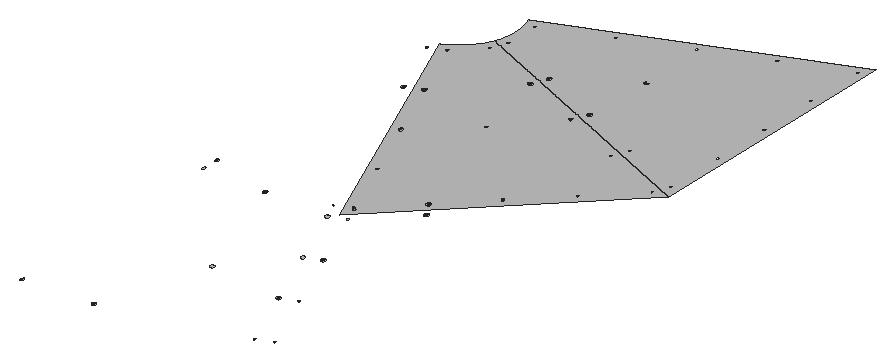
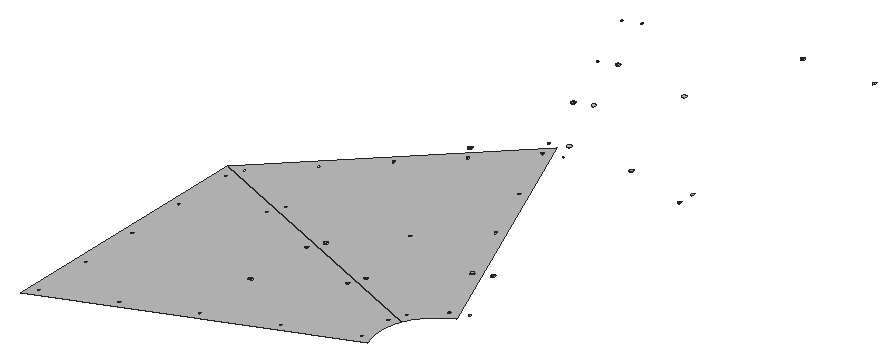
# SketchUp Ruby script. Lengths in inches.
U = 1.inch
M = Sketchup.active_model
def pt(a) = Geom::Point3d.new(a.map { |v| v * U })
def face(e, loops, mat)
  f = e.add_face(loops[0].map { |a| pt(a) })
  loops[1..].each { |l| e.add_face(l.map { |a| pt(a) }).erase! }
  f.material = f.back_material = mat if mat
  f
end
# faces: each face lists its corners as indices into pts; further lists are holes
def faces(e, pts, list, mat = nil) = list.each { |f| face(e, (f[0].is_a?(Array) ? f : [f]).map { |l| l.map { |i| pts[i] } }, mat) }
# xy, xz, yz: faces in a plane at the given z, y or x. An outline is a flat list of corners, or four numbers for a rectangle; further outlines are holes
def ring(l) = l.size == 4 ? [[l[0], l[1]], [l[2], l[1]], [l[2], l[3]], [l[0], l[3]]] : l.each_slice(2).to_a
def flat(e, list, mat, &to3) = list.each { |f| face(e, (f[0].is_a?(Array) ? f : [f]).map { |l| ring(l).map { |u, v| to3.(u, v) } }, mat) }
def xy(e, z, list, mat = nil) = flat(e, list, mat) { |x, y| [x, y, z] }
def xz(e, y, list, mat = nil) = flat(e, list, mat) { |x, z| [x, y, z] }
def yz(e, x, list, mat = nil) = flat(e, list, mat) { |y, z| [x, y, z] }
def lines(e, pts, list) = list.each { |a, b| e.add_line(pt(pts[a]), pt(pts[b])) }
# prism: a flat outline (further loops are holes) pulled along v
def prism(e, loops, v, mat = nil)
  f = face(e, loops, mat); d = Geom::Vector3d.new(v.map { |x| x * U })
  f.pushpull(f.normal.samedirection?(d) ? d.length : -d.length)
end
def box(e, o, s, mat = nil) = prism(e, [[o, [o[0] + s[0], o[1], o[2]], [o[0] + s[0], o[1] + s[1], o[2]], [o[0], o[1] + s[1], o[2]]]], [0, 0, s[2]], mat)
def at(x, y, z, deg = 0) = Geom::Transformation.translation(pt([x, y, z])) * Geom::Transformation.rotation(ORIGIN, Z_AXIS, deg.degrees)
def axes(o, x, y, z) = Geom::Transformation.new([*x, 0, *y, 0, *z, 0, *pt(o).to_a, 1])
def part(name) = M.definitions.add(name)
# library, detail: a bought-in or finely detailed component or shape, given as its bounding box
def library(name, o, s) = part(name).tap { |d| box(d.entities, o, s) }
def detail(e, o, s) = box(e.add_group.entities, o, s)
def put(e, d, t, mat = nil) = e.add_instance(d, t).tap { |i| i.material = mat if mat }
def group(e, t, mat = nil) = e.add_group.tap { |g| g.transformation = t; g.material = mat if mat }.entities
root = M.entities
M.materials.add("[Metal_Steel_Textured_White]").color = [191, 191, 191]
xy(root,3.625,[[149.818,137.074,149.818,137.125,149.827,137.127,149.836,137.13,149.844,137.136,149.85,137.144,149.853,137.153,149.854,137.162,149.853,137.172,149.85,137.18,149.844,137.188,149.836,137.194,149.827,137.197,149.818,137.199,149.818,137.25,149.841,137.247,149.862,137.238,149.88,137.224,149.894,137.206,149.903,137.185,149.906,137.162,149.903,137.139,149.894,137.118,149.88,137.1,149.862,137.086,149.841,137.077],[149.818,137.125,149.818,137.142,149.823,137.143,149.828,137.145,149.832,137.148,149.835,137.152,149.837,137.157,149.838,137.162,149.837,137.167,149.835,137.172,149.832,137.176,149.828,137.179,149.823,137.181,149.818,137.182,149.818,137.199,149.827,137.197,149.836,137.194,149.844,137.188,149.85,137.18,149.853,137.172,149.854,137.162,149.853,137.153,149.85,137.144,149.844,137.136,149.836,137.13,149.827,137.127],[[153.108,137.28,153.085,137.283,153.063,137.292,153.045,137.306,153.031,137.325,153.022,137.346,153.019,137.369,153.022,137.392,153.031,137.414,153.045,137.432,153.063,137.446,153.085,137.455,153.108,137.458,153.131,137.455,153.152,137.446,153.171,137.432,153.185,137.414,153.194,137.392,153.197,137.369,153.194,137.346,153.185,137.325,153.171,137.306,153.152,137.292,153.131,137.283],[153.108,137.281,153.13,137.284,153.152,137.293,153.17,137.307,153.184,137.325,153.193,137.347,153.196,137.369,153.193,137.392,153.184,137.413,153.17,137.432,153.152,137.445,153.13,137.454,153.108,137.457,153.085,137.454,153.064,137.445,153.046,137.432,153.032,137.413,153.023,137.392,153.02,137.369,153.023,137.347,153.032,137.325,153.046,137.307,153.064,137.293,153.085,137.284]],[[153.108,137.281,153.085,137.284,153.064,137.293,153.046,137.307,153.032,137.325,153.023,137.347,153.02,137.369,153.023,137.392,153.032,137.413,153.046,137.432,153.064,137.445,153.085,137.454,153.108,137.457,153.13,137.454,153.152,137.445,153.17,137.432,153.184,137.413,153.193,137.392,153.196,137.369,153.193,137.347,153.184,137.325,153.17,137.307,153.152,137.293,153.13,137.284],[153.108,137.333,153.117,137.334,153.126,137.338,153.134,137.343,153.139,137.351,153.143,137.36,153.144,137.369,153.143,137.379,153.139,137.388,153.134,137.395,153.126,137.401,153.117,137.405,153.108,137.406,153.098,137.405,153.089,137.401,153.082,137.395,153.076,137.388,153.072,137.379,153.071,137.369,153.072,137.36,153.076,137.351,153.082,137.343,153.089,137.338,153.098,137.334]],[[159.48,138.971,159.471,138.972,159.462,138.976,159.454,138.982,159.448,138.989,159.445,138.998,159.443,139.008,159.445,139.017,159.448,139.026,159.454,139.034,159.462,139.039,159.471,139.043,159.48,139.044,159.49,139.043,159.498,139.039,159.506,139.034,159.512,139.026,159.515,139.017,159.517,139.008,159.515,138.998,159.512,138.989,159.506,138.982,159.498,138.976,159.49,138.972],[159.475,138.988,159.485,138.988,159.49,138.99,159.494,138.994,159.497,138.998,159.499,139.002,159.5,139.008,159.499,139.013,159.497,139.018,159.494,139.022,159.49,139.025,159.485,139.027,159.48,139.028,159.475,139.027,159.47,139.025,159.466,139.022,159.463,139.018,159.461,139.013,159.46,139.008,159.461,139.002,159.463,138.998,159.466,138.994,159.47,138.99]],
  [159.475,138.988,159.47,138.99,159.466,138.994,159.463,138.998,159.461,139.002,159.46,139.008,159.461,139.013,159.463,139.018,159.466,139.022,159.47,139.025,159.475,139.027,159.48,139.028,159.485,139.027,159.49,139.025,159.494,139.022,159.497,139.018,159.499,139.013,159.5,139.008,159.499,139.002,159.497,138.998,159.494,138.994,159.49,138.99,159.485,138.988],[[160.218,139.277,160.208,139.278,160.199,139.282,160.192,139.287,160.186,139.295,160.182,139.304,160.181,139.313,160.182,139.323,160.186,139.331,160.192,139.339,160.199,139.345,160.208,139.349,160.218,139.35,160.227,139.349,160.236,139.345,160.244,139.339,160.249,139.331,160.253,139.323,160.254,139.313,160.253,139.304,160.249,139.295,160.244,139.287,160.236,139.282,160.227,139.278],[160.218,139.293,160.223,139.294,160.228,139.296,160.232,139.299,160.235,139.303,160.237,139.308,160.238,139.313,160.237,139.318,160.235,139.323,160.232,139.327,160.228,139.33,160.223,139.332,160.218,139.333,160.213,139.332,160.208,139.33,160.204,139.327,160.2,139.323,160.198,139.318,160.198,139.308,160.2,139.303,160.204,139.299,160.208,139.296,160.213,139.294]],[160.218,139.293,160.213,139.294,160.208,139.296,160.204,139.299,160.2,139.303,160.198,139.308,160.198,139.318,160.2,139.323,160.204,139.327,160.208,139.33,160.213,139.332,160.218,139.333,160.223,139.332,160.228,139.33,160.232,139.327,160.235,139.323,160.237,139.318,160.238,139.313,160.237,139.308,160.235,139.303,160.232,139.299,160.228,139.296,160.223,139.294],[[158.237,141.919,158.214,141.922,158.193,141.931,158.175,141.945,158.16,141.963,158.152,141.985,158.149,142.008,158.152,142.031,158.16,142.052,158.175,142.07,158.193,142.085,158.214,142.093,158.237,142.096,158.26,142.093,158.282,142.085,158.3,142.07,158.314,142.052,158.323,142.031,158.326,142.008,158.323,141.985,158.314,141.963,158.3,141.945,158.282,141.931,158.26,141.922],[158.237,141.92,158.26,141.923,158.281,141.931,158.3,141.945,158.314,141.964,158.322,141.985,158.325,142.008,158.322,142.03,158.314,142.052,158.3,142.07,158.281,142.084,158.26,142.093,158.237,142.096,158.215,142.093,158.193,142.084,158.175,142.07,158.161,142.052,158.153,142.03,158.15,142.008,158.153,141.985,158.161,141.964,158.175,141.945,158.193,141.931,158.215,141.923]],[[158.237,141.971,158.228,141.972,158.219,141.976,158.212,141.982,158.206,141.989,158.202,141.998,158.201,142.008,158.202,142.017,158.206,142.026,158.212,142.033,158.219,142.039,158.228,142.043,158.237,142.044,158.247,142.043,158.256,142.039,158.263,142.033,158.269,142.026,158.273,142.017,158.274,142.008,158.273,141.998,158.269,141.989,158.263,141.982,158.256,141.976,158.247,141.972],[158.232,141.988,158.243,141.988,158.247,141.99,158.252,141.993,158.255,141.998,158.257,142.002,158.257,142.013,158.255,142.018,158.252,142.022,158.247,142.025,158.243,142.027,158.237,142.028,158.232,142.027,158.227,142.025,158.223,142.022,158.22,142.018,158.218,142.013,158.217,142.008,158.218,142.002,158.22,141.998,158.223,141.993,158.227,141.99]],
  [158.232,141.988,158.227,141.99,158.223,141.993,158.22,141.998,158.218,142.002,158.217,142.008,158.218,142.013,158.22,142.018,158.223,142.022,158.227,142.025,158.232,142.027,158.237,142.028,158.243,142.027,158.247,142.025,158.252,142.022,158.255,142.018,158.257,142.013,158.257,142.002,158.255,141.998,158.252,141.993,158.247,141.99,158.243,141.988],[[154.784,142.264,154.761,142.267,154.74,142.276,154.722,142.29,154.708,142.308,154.699,142.329,154.696,142.352,154.699,142.375,154.708,142.396,154.722,142.414,154.74,142.428,154.761,142.437,154.784,142.44,154.807,142.437,154.828,142.428,154.846,142.414,154.86,142.396,154.869,142.375,154.872,142.352,154.869,142.329,154.86,142.308,154.846,142.29,154.828,142.276,154.807,142.267],[154.784,142.315,154.794,142.317,154.802,142.32,154.81,142.326,154.816,142.334,154.819,142.342,154.821,142.352,154.819,142.361,154.816,142.37,154.81,142.378,154.802,142.384,154.794,142.387,154.784,142.389,154.775,142.387,154.766,142.384,154.758,142.378,154.752,142.37,154.749,142.361,154.747,142.352,154.749,142.342,154.752,142.334,154.758,142.326,154.766,142.32,154.775,142.317]],[[158.975,142.277,158.966,142.278,158.957,142.281,158.949,142.287,158.943,142.295,158.94,142.304,158.939,142.313,158.94,142.323,158.943,142.331,158.949,142.339,158.957,142.345,158.966,142.349,158.975,142.35,158.985,142.349,158.993,142.345,159.001,142.339,159.007,142.331,159.01,142.323,159.012,142.313,159.01,142.304,159.007,142.295,159.001,142.287,158.993,142.281,158.985,142.278],[158.975,142.293,158.98,142.294,158.985,142.296,158.989,142.299,158.992,142.303,158.994,142.308,158.995,142.313,158.994,142.318,158.992,142.323,158.989,142.327,158.985,142.33,158.98,142.332,158.975,142.333,158.97,142.332,158.965,142.33,158.961,142.327,158.958,142.323,158.956,142.318,158.955,142.313,158.956,142.308,158.958,142.303,158.961,142.299,158.965,142.296,158.97,142.294]],[158.975,142.293,158.97,142.294,158.965,142.296,158.961,142.299,158.958,142.303,158.956,142.308,158.955,142.313,158.956,142.318,158.958,142.323,158.961,142.327,158.965,142.33,158.97,142.332,158.975,142.333,158.98,142.332,158.985,142.33,158.989,142.327,158.992,142.323,158.994,142.318,158.995,142.313,158.994,142.308,158.992,142.303,158.989,142.299,158.985,142.296,158.98,142.294],[[156.995,144.92,156.972,144.923,156.951,144.931,156.933,144.945,156.919,144.964,156.91,144.985,156.907,145.008,156.91,145.03,156.919,145.052,156.933,145.07,156.951,145.084,156.972,145.092,156.995,145.095,157.018,145.092,157.039,145.084,157.057,145.07,157.071,145.052,157.08,145.03,157.083,145.008,157.08,144.985,157.071,144.964,157.057,144.945,157.039,144.931,157.018,144.923],[156.995,144.971,157.004,144.972,157.013,144.976,157.021,144.982,157.027,144.989,157.03,144.998,157.031,145.008,157.03,145.017,157.027,145.026,157.021,145.033,157.013,145.039,157.004,145.043,156.995,145.044,156.985,145.043,156.977,145.039,156.969,145.033,156.963,145.026,156.959,145.017,156.958,145.008,156.959,144.998,156.963,144.989,156.969,144.982,156.977,144.976,156.985,144.972]],
  [[157.732,145.224,157.709,145.227,157.688,145.236,157.67,145.25,157.656,145.269,157.647,145.29,157.644,145.313,157.647,145.336,157.656,145.358,157.67,145.376,157.688,145.39,157.709,145.399,157.732,145.402,157.755,145.399,157.777,145.39,157.795,145.376,157.809,145.358,157.818,145.336,157.821,145.313,157.818,145.29,157.809,145.269,157.795,145.25,157.777,145.236,157.755,145.227],[157.732,145.225,157.755,145.228,157.776,145.237,157.795,145.251,157.809,145.269,157.817,145.29,157.82,145.313,157.817,145.336,157.809,145.357,157.795,145.375,157.776,145.389,157.755,145.398,157.732,145.401,157.71,145.398,157.689,145.389,157.67,145.375,157.656,145.357,157.648,145.336,157.645,145.313,157.648,145.29,157.656,145.269,157.67,145.251,157.689,145.237,157.71,145.228]],[[157.732,145.277,157.723,145.278,157.714,145.281,157.707,145.287,157.701,145.295,157.697,145.304,157.696,145.313,157.697,145.323,157.701,145.331,157.707,145.339,157.714,145.345,157.723,145.348,157.732,145.35,157.742,145.348,157.751,145.345,157.758,145.339,157.764,145.331,157.768,145.323,157.769,145.313,157.768,145.304,157.764,145.295,157.758,145.287,157.751,145.281,157.742,145.278],[157.732,145.293,157.738,145.294,157.742,145.296,157.747,145.299,157.75,145.303,157.752,145.308,157.752,145.318,157.75,145.323,157.747,145.327,157.742,145.33,157.738,145.332,157.732,145.333,157.727,145.332,157.723,145.33,157.718,145.327,157.715,145.323,157.713,145.318,157.713,145.308,157.715,145.303,157.718,145.299,157.723,145.296,157.727,145.294]],[157.732,145.293,157.727,145.294,157.723,145.296,157.718,145.299,157.715,145.303,157.713,145.308,157.713,145.318,157.715,145.323,157.718,145.327,157.723,145.33,157.727,145.332,157.732,145.333,157.738,145.332,157.742,145.33,157.747,145.327,157.75,145.323,157.752,145.318,157.752,145.308,157.75,145.303,157.747,145.299,157.742,145.296,157.738,145.294],[[152.785,147.919,152.762,147.922,152.741,147.931,152.722,147.945,152.708,147.963,152.699,147.985,152.696,148.008,152.699,148.031,152.708,148.052,152.722,148.07,152.741,148.085,152.762,148.093,152.785,148.096,152.808,148.093,152.829,148.085,152.848,148.07,152.862,148.052,152.871,148.031,152.874,148.008,152.871,147.985,152.862,147.963,152.848,147.945,152.829,147.931,152.808,147.922],[152.785,147.92,152.808,147.923,152.829,147.931,152.847,147.945,152.861,147.964,152.87,147.985,152.873,148.008,152.87,148.03,152.861,148.051,152.847,148.07,152.829,148.084,152.808,148.092,152.785,148.095,152.762,148.092,152.741,148.084,152.723,148.07,152.709,148.051,152.7,148.03,152.697,148.008,152.7,147.985,152.709,147.964,152.723,147.945,152.741,147.931,152.762,147.923]],[[155.752,147.919,155.729,147.922,155.708,147.931,155.689,147.945,155.675,147.963,155.666,147.985,155.663,148.008,155.666,148.031,155.675,148.052,155.689,148.07,155.708,148.085,155.729,148.093,155.752,148.096,155.775,148.093,155.797,148.085,155.815,148.07,155.829,148.052,155.838,148.031,155.841,148.008,155.838,147.985,155.829,147.963,155.815,147.945,155.797,147.931,155.775,147.922],[155.752,147.92,155.775,147.923,155.796,147.931,155.814,147.945,155.828,147.964,155.837,147.985,155.84,148.008,155.837,148.03,155.828,148.051,155.814,148.07,155.796,148.084,155.775,148.092,155.752,148.095,155.729,148.092,155.708,148.084,155.69,148.07,155.676,148.051,155.667,148.03,155.664,148.008,155.667,147.985,155.676,147.964,155.69,147.945,155.708,147.931,155.729,147.923]],
  [149.818,147.92,149.818,147.971,149.827,147.972,149.836,147.976,149.844,147.982,149.85,147.989,149.853,147.998,149.854,148.008,149.853,148.017,149.85,148.026,149.844,148.033,149.836,148.039,149.827,148.043,149.818,148.044,149.818,148.095,149.841,148.092,149.862,148.084,149.88,148.07,149.894,148.051,149.903,148.03,149.906,148.008,149.903,147.985,149.894,147.964,149.88,147.945,149.862,147.931,149.841,147.923],[[152.785,147.92,152.762,147.923,152.741,147.931,152.723,147.945,152.709,147.964,152.7,147.985,152.697,148.008,152.7,148.03,152.709,148.051,152.723,148.07,152.741,148.084,152.762,148.092,152.785,148.095,152.808,148.092,152.829,148.084,152.847,148.07,152.861,148.051,152.87,148.03,152.873,148.008,152.87,147.985,152.861,147.964,152.847,147.945,152.829,147.931,152.808,147.923],[152.785,147.971,152.795,147.972,152.803,147.976,152.811,147.982,152.817,147.989,152.82,147.998,152.822,148.008,152.82,148.017,152.817,148.026,152.811,148.033,152.803,148.039,152.795,148.043,152.785,148.044,152.776,148.043,152.767,148.039,152.759,148.033,152.753,148.026,152.75,148.017,152.748,148.008,152.75,147.998,152.753,147.989,152.759,147.982,152.767,147.976,152.776,147.972]],[[155.752,147.92,155.729,147.923,155.708,147.931,155.69,147.945,155.676,147.964,155.667,147.985,155.664,148.008,155.667,148.03,155.676,148.051,155.69,148.07,155.708,148.084,155.729,148.092,155.752,148.095,155.775,148.092,155.796,148.084,155.814,148.07,155.828,148.051,155.837,148.03,155.84,148.008,155.837,147.985,155.828,147.964,155.814,147.945,155.796,147.931,155.775,147.923],[155.752,147.971,155.762,147.972,155.771,147.976,155.778,147.982,155.784,147.989,155.788,147.998,155.789,148.008,155.788,148.017,155.784,148.026,155.778,148.033,155.771,148.039,155.762,148.043,155.752,148.044,155.743,148.043,155.734,148.039,155.726,148.033,155.721,148.026,155.717,148.017,155.716,148.008,155.717,147.998,155.721,147.989,155.726,147.982,155.734,147.976,155.743,147.972]],[[156.49,148.276,156.48,148.278,156.472,148.281,156.464,148.287,156.458,148.295,156.455,148.304,156.453,148.313,156.455,148.323,156.458,148.331,156.464,148.339,156.472,148.345,156.48,148.348,156.49,148.35,156.499,148.348,156.508,148.345,156.516,148.339,156.522,148.331,156.525,148.323,156.526,148.313,156.525,148.304,156.522,148.295,156.516,148.287,156.508,148.281,156.499,148.278],[156.49,148.293,156.495,148.294,156.5,148.296,156.504,148.299,156.507,148.303,156.509,148.308,156.51,148.313,156.509,148.318,156.507,148.323,156.504,148.327,156.5,148.33,156.495,148.332,156.49,148.333,156.485,148.332,156.48,148.33,156.476,148.327,156.473,148.323,156.471,148.318,156.47,148.313,156.471,148.308,156.473,148.303,156.476,148.299,156.48,148.296,156.485,148.294]],[156.49,148.293,156.485,148.294,156.48,148.296,156.476,148.299,156.473,148.303,156.471,148.308,156.47,148.313,156.471,148.318,156.473,148.323,156.476,148.327,156.48,148.33,156.485,148.332,156.49,148.333,156.495,148.332,156.5,148.33,156.504,148.327,156.507,148.323,156.509,148.318,156.51,148.313,156.509,148.308,156.507,148.303,156.504,148.299,156.5,148.296,156.495,148.294],
  [[156.019,148.407,150.836,160.919,150.995,160.99,151.149,161.073,151.297,161.165,151.438,161.266,151.573,161.376,151.7,161.495,151.819,161.623,151.929,161.757,152.031,161.899,152.123,162.047,152.205,162.2,152.277,162.359,164.789,157.176],[152.551,157.734,152.574,157.737,152.595,157.746,152.614,157.76,152.628,157.778,152.637,157.8,152.64,157.823,152.637,157.846,152.628,157.867,152.614,157.886,152.595,157.9,152.574,157.909,152.551,157.912,152.528,157.909,152.506,157.9,152.488,157.886,152.474,157.867,152.465,157.846,152.462,157.823,152.465,157.8,152.474,157.778,152.488,157.76,152.506,157.746,152.528,157.737],[164.084,156.947,164.107,156.95,164.128,156.959,164.147,156.973,164.161,156.992,164.17,157.013,164.173,157.036,164.17,157.059,164.161,157.081,164.147,157.099,164.128,157.113,164.107,157.122,164.084,157.125,164.061,157.122,164.039,157.113,164.021,157.099,164.007,157.081,163.998,157.059,163.995,157.036,163.998,157.013,164.007,156.992,164.021,156.973,164.039,156.959,164.061,156.95],[158.14,151.004,158.163,151.007,158.185,151.016,158.203,151.03,158.217,151.048,158.226,151.07,158.229,151.093,158.226,151.116,158.217,151.137,158.203,151.156,158.185,151.17,158.163,151.179,158.14,151.182,158.117,151.179,158.096,151.17,158.077,151.156,158.063,151.137,158.054,151.116,158.051,151.093,158.054,151.07,158.063,151.048,158.077,151.03,158.096,151.016,158.117,151.007],[156.122,156.984,156.145,156.987,156.167,156.996,156.185,157.01,156.199,157.029,156.208,157.05,156.211,157.073,156.208,157.096,156.199,157.117,156.185,157.136,156.167,157.15,156.145,157.159,156.122,157.162,156.099,157.159,156.078,157.15,156.06,157.136,156.045,157.117,156.037,157.096,156.033,157.073,156.037,157.05,156.045,157.029,156.06,157.01,156.078,156.996,156.099,156.987],[155.372,160.556,155.395,160.559,155.417,160.568,155.435,160.582,155.449,160.6,155.458,160.622,155.461,160.645,155.458,160.668,155.449,160.689,155.435,160.707,155.417,160.722,155.395,160.73,155.372,160.733,155.349,160.73,155.328,160.722,155.31,160.707,155.295,160.689,155.287,160.668,155.284,160.645,155.287,160.622,155.295,160.6,155.31,160.582,155.328,160.568,155.349,160.559],[158.276,159.353,158.299,159.356,158.321,159.365,158.339,159.379,158.353,159.397,158.362,159.419,158.365,159.442,158.362,159.465,158.353,159.486,158.339,159.505,158.321,159.519,158.299,159.528,158.276,159.531,158.253,159.528,158.232,159.519,158.213,159.505,158.199,159.486,158.19,159.465,158.1875,159.442,158.19,159.419,158.199,159.397,158.213,159.379,158.232,159.365,158.253,159.356],[156.159,149.023,156.182,149.026,156.204,149.035,156.222,149.049,156.236,149.067,156.245,149.088,156.248,149.112,156.245,149.135,156.236,149.156,156.222,149.174,156.204,149.188,156.182,149.197,156.159,149.2,156.136,149.197,156.115,149.188,156.096,149.174,156.082,149.156,156.073,149.135,156.07,149.112,156.073,149.088,156.082,149.067,156.096,149.049,156.115,149.035,156.136,149.026],[162.103,154.966,162.126,154.969,162.147,154.978,162.165,154.992,162.18,155.011,162.189,155.032,162.192,155.055,162.189,155.078,162.18,155.099,162.165,155.118,162.147,155.132,162.126,155.141,162.103,155.144,162.08,155.141,162.058,155.132,162.04,155.118,162.026,155.099,162.017,155.078,162.014,155.055,162.017,155.032,162.026,155.011,162.04,154.992,162.058,154.978,162.08,154.969],[152.469,161.758,152.492,161.761,152.513,161.77,152.532,161.784,152.546,161.803,152.555,161.824,152.558,161.847,152.555,161.87,152.546,161.892,152.532,161.91,152.513,161.924,152.492,161.933,152.469,161.936,152.446,161.933,152.424,161.924,152.406,161.91,152.392,161.892,152.383,161.87,152.38,161.847,152.383,161.824,152.392,161.803,152.406,161.784,152.424,161.77,152.446,161.761],[161.18,158.15,161.203,158.153,161.224,158.162,161.243,158.176,161.257,158.195,161.266,158.216,161.269,158.239,161.266,158.262,161.257,158.283,161.243,158.302,161.224,158.316,161.203,158.325,161.18,158.328,161.157,158.325,161.136,158.316,161.117,158.302,161.103,158.283,161.094,158.262,161.091,158.239,161.094,158.216,161.103,158.195,161.117,158.176,161.136,158.162,161.157,158.153],[154.956,151.926,154.979,151.929,155.001,151.938,155.019,151.952,155.033,151.971,155.042,151.992,155.045,152.015,155.042,152.038,155.033,152.06,155.019,152.078,155.001,152.092,154.979,152.101,154.956,152.104,154.933,152.101,154.912,152.092,154.893,152.078,154.879,152.06,154.87,152.038,154.867,152.015,154.87,151.992,154.879,151.971,154.893,151.952,154.912,151.938,154.933,151.929],[160.121,152.985,160.144,152.988,160.166,152.997,160.184,153.011,160.198,153.029,160.207,153.051,160.21,153.074,160.207,153.097,160.198,153.118,160.184,153.137,160.166,153.151,160.144,153.16,160.121,153.163,160.098,153.16,160.077,153.151,160.059,153.137,160.044,153.118,160.036,153.097,160.033,153.074,160.036,153.051,160.044,153.029,160.059,153.011,160.077,152.997,160.098,152.988],[151.348,160.638,151.371,160.641,151.392,160.65,151.411,160.664,151.425,160.682,151.434,160.704,151.437,160.727,151.434,160.75,151.425,160.771,151.411,160.79,151.392,160.804,151.371,160.8125,151.348,160.816,151.325,160.8125,151.304,160.804,151.285,160.79,151.271,160.771,151.262,160.75,151.259,160.727,151.262,160.704,151.271,160.682,151.285,160.664,151.304,160.65,151.325,160.641],[153.754,154.83,153.777,154.833,153.798,154.842,153.816,154.856,153.831,154.875,153.839,154.896,153.842,154.919,153.839,154.942,153.831,154.964,153.816,154.982,153.798,154.996,153.777,155.005,153.754,155.008,153.731,155.005,153.709,154.996,153.691,154.982,153.677,154.964,153.668,154.942,153.665,154.919,153.668,154.896,153.677,154.875,153.691,154.856,153.709,154.842,153.731,154.833]],[149.818,148.718,149.818,148.769,149.827,148.771,149.836,148.774,149.844,148.78,149.85,148.788,149.853,148.796,149.854,148.806,149.853,148.815,149.85,148.824,149.844,148.832,149.836,148.838,149.827,148.841,149.818,148.843,149.818,148.894,149.841,148.891,149.862,148.882,149.88,148.868,149.894,148.85,149.903,148.829,149.906,148.806,149.903,148.783,149.894,148.762,149.88,148.744,149.862,148.73,149.841,148.721],[149.818,148.769,149.818,148.786,149.823,148.787,149.828,148.789,149.832,148.792,149.835,148.796,149.837,148.801,149.838,148.806,149.837,148.811,149.835,148.816,149.832,148.82,149.828,148.823,149.823,148.825,149.818,148.826,149.818,148.843,149.827,148.841,149.836,148.838,149.844,148.832,149.85,148.824,149.853,148.815,149.854,148.806,149.853,148.796,149.85,148.788,149.844,148.78,149.836,148.774,149.827,148.771],[149.818,148.786,149.818,148.826,149.823,148.825,149.828,148.823,149.832,148.82,149.835,148.816,149.837,148.811,149.838,148.806,149.837,148.801,149.835,148.796,149.832,148.792,149.828,148.789,149.823,148.787],[155.421,148.786,155.416,148.787,155.412,148.789,155.407,148.792,155.404,148.796,155.402,148.801,155.402,148.811,155.404,148.816,155.407,148.82,155.412,148.823,155.416,148.825,155.421,148.826,155.427,148.825,155.431,148.823,155.436,148.82,155.439,148.816,155.441,148.811,155.441,148.801,155.439,148.796,155.436,148.792,155.431,148.789,155.427,148.787],
  [[156.159,149.023,156.136,149.026,156.115,149.035,156.096,149.049,156.082,149.067,156.073,149.088,156.07,149.112,156.073,149.135,156.082,149.156,156.096,149.174,156.115,149.188,156.136,149.197,156.159,149.2,156.182,149.197,156.204,149.188,156.222,149.174,156.236,149.156,156.245,149.135,156.248,149.112,156.245,149.088,156.236,149.067,156.222,149.049,156.204,149.035,156.182,149.026],[156.159,149.024,156.182,149.027,156.203,149.035,156.221,149.049,156.235,149.068,156.244,149.089,156.247,149.112,156.244,149.134,156.235,149.155,156.221,149.174,156.203,149.1875,156.182,149.196,156.159,149.199,156.136,149.196,156.115,149.1875,156.097,149.174,156.083,149.155,156.074,149.134,156.071,149.112,156.074,149.089,156.083,149.068,156.097,149.049,156.115,149.035,156.136,149.027]],[[156.159,149.075,156.15,149.076,156.141,149.08,156.133,149.086,156.127,149.093,156.124,149.102,156.123,149.112,156.124,149.121,156.127,149.13,156.133,149.137,156.141,149.143,156.15,149.147,156.159,149.148,156.169,149.147,156.177,149.143,156.185,149.137,156.191,149.13,156.194,149.121,156.196,149.112,156.194,149.102,156.191,149.093,156.185,149.086,156.177,149.08,156.169,149.076],[156.154,149.092,156.164,149.092,156.169,149.094,156.173,149.097,156.176,149.102,156.178,149.106,156.179,149.112,156.178,149.117,156.176,149.121,156.173,149.126,156.169,149.129,156.164,149.131,156.154,149.131,156.149,149.129,156.145,149.126,156.142,149.121,156.14,149.117,156.139,149.112,156.14,149.106,156.142,149.102,156.145,149.097,156.149,149.094]],[156.154,149.092,156.149,149.094,156.145,149.097,156.142,149.102,156.14,149.106,156.139,149.112,156.14,149.117,156.142,149.121,156.145,149.126,156.149,149.129,156.154,149.131,156.164,149.131,156.169,149.129,156.173,149.126,156.176,149.121,156.178,149.117,156.179,149.112,156.178,149.106,156.176,149.102,156.173,149.097,156.169,149.094,156.164,149.092],[[158.588,150.322,158.565,150.325,158.544,150.334,158.525,150.348,158.511,150.367,158.502,150.388,158.499,150.411,158.502,150.434,158.511,150.456,158.525,150.474,158.544,150.488,158.565,150.497,158.588,150.5,158.611,150.497,158.632,150.488,158.651,150.474,158.665,150.456,158.674,150.434,158.677,150.411,158.674,150.388,158.665,150.367,158.651,150.348,158.632,150.334,158.611,150.325],[158.588,150.323,158.611,150.326,158.632,150.335,158.65,150.349,158.664,150.367,158.673,150.388,158.676,150.411,158.673,150.434,158.664,150.455,158.65,150.473,158.632,150.487,158.611,150.496,158.588,150.499,158.565,150.496,158.544,150.487,158.526,150.473,158.512,150.455,158.503,150.434,158.5,150.411,158.503,150.388,158.512,150.367,158.526,150.349,158.544,150.335,158.565,150.326]],[[158.588,150.375,158.578,150.376,158.57,150.379,158.562,150.385,158.556,150.393,158.553,150.402,158.551,150.411,158.553,150.421,158.556,150.429,158.562,150.437,158.57,150.443,158.578,150.447,158.588,150.448,158.597,150.447,158.606,150.443,158.614,150.437,158.62,150.429,158.623,150.421,158.625,150.411,158.623,150.402,158.62,150.393,158.614,150.385,158.606,150.379,158.597,150.376],[158.588,150.391,158.593,150.392,158.598,150.394,158.602,150.397,158.605,150.401,158.607,150.406,158.608,150.411,158.607,150.416,158.605,150.421,158.602,150.425,158.598,150.428,158.593,150.43,158.588,150.431,158.583,150.43,158.578,150.428,158.574,150.425,158.571,150.421,158.569,150.416,158.568,150.411,158.569,150.406,158.571,150.401,158.574,150.397,158.578,150.394,158.583,150.392]],
  [158.588,150.391,158.583,150.392,158.578,150.394,158.574,150.397,158.571,150.401,158.569,150.406,158.568,150.411,158.569,150.416,158.571,150.421,158.574,150.425,158.578,150.428,158.583,150.43,158.588,150.431,158.593,150.43,158.598,150.428,158.602,150.425,158.605,150.421,158.607,150.416,158.608,150.411,158.607,150.406,158.605,150.401,158.602,150.397,158.598,150.394,158.593,150.392],[[158.14,151.004,158.117,151.007,158.096,151.016,158.077,151.03,158.063,151.048,158.054,151.07,158.051,151.093,158.054,151.116,158.063,151.137,158.077,151.156,158.096,151.17,158.117,151.179,158.14,151.182,158.163,151.179,158.185,151.17,158.203,151.156,158.217,151.137,158.226,151.116,158.229,151.093,158.226,151.07,158.217,151.048,158.203,151.03,158.185,151.016,158.163,151.007],[158.14,151.005,158.163,151.008,158.184,151.017,158.202,151.03,158.216,151.049,158.225,151.07,158.228,151.093,158.225,151.115,158.216,151.137,158.202,151.155,158.184,151.169,158.163,151.178,158.14,151.181,158.118,151.178,158.096,151.169,158.078,151.155,158.064,151.137,158.055,151.115,158.052,151.093,158.055,151.07,158.064,151.049,158.078,151.03,158.096,151.017,158.118,151.008]],[[158.14,151.056,158.131,151.057,158.122,151.061,158.114,151.067,158.109,151.074,158.105,151.083,158.104,151.093,158.105,151.102,158.109,151.111,158.114,151.119,158.122,151.124,158.131,151.128,158.14,151.129,158.15,151.128,158.159,151.124,158.166,151.119,158.172,151.111,158.176,151.102,158.177,151.093,158.176,151.083,158.172,151.074,158.166,151.067,158.159,151.061,158.15,151.057],[158.135,151.073,158.145,151.073,158.15,151.075,158.158,151.083,158.16,151.088,158.16,151.098,158.158,151.103,158.154,151.107,158.15,151.11,158.145,151.112,158.14,151.113,158.135,151.112,158.13,151.11,158.126,151.107,158.123,151.103,158.121,151.098,158.12,151.093,158.121,151.088,158.123,151.083,158.126,151.079,158.13,151.075]],[158.135,151.073,158.13,151.075,158.126,151.079,158.123,151.083,158.121,151.088,158.12,151.093,158.121,151.098,158.123,151.103,158.126,151.107,158.13,151.11,158.135,151.112,158.14,151.113,158.145,151.112,158.15,151.11,158.154,151.107,158.158,151.103,158.16,151.098,158.16,151.088,158.158,151.083,158.15,151.075,158.145,151.073],[[154.956,151.979,154.947,151.98,154.938,151.984,154.93,151.989,154.925,151.997,154.921,152.006,154.92,152.015,154.921,152.025,154.925,152.034,154.93,152.041,154.938,152.047,154.947,152.051,154.956,152.052,154.966,152.051,154.975,152.047,154.982,152.041,154.988,152.034,154.992,152.025,154.993,152.015,154.992,152.006,154.988,151.997,154.982,151.989,154.975,151.984,154.966,151.98],[154.956,151.995,154.962,151.996,154.966,151.998,154.97,152.001,154.974,152.005,154.976,152.01,154.976,152.02,154.974,152.025,154.966,152.033,154.962,152.035,154.951,152.035,154.946,152.033,154.942,152.029,154.939,152.025,154.937,152.02,154.936,152.015,154.937,152.01,154.939,152.005,154.942,152.001,154.946,151.998,154.951,151.996]],
  [154.956,151.995,154.951,151.996,154.946,151.998,154.942,152.001,154.939,152.005,154.937,152.01,154.936,152.015,154.937,152.02,154.939,152.025,154.942,152.029,154.946,152.033,154.951,152.035,154.962,152.035,154.966,152.033,154.974,152.025,154.976,152.02,154.976,152.01,154.974,152.005,154.97,152.001,154.966,151.998,154.962,151.996],[[160.121,152.985,160.098,152.988,160.077,152.997,160.059,153.011,160.044,153.029,160.036,153.051,160.033,153.074,160.036,153.097,160.044,153.118,160.059,153.137,160.077,153.151,160.098,153.16,160.121,153.163,160.144,153.16,160.166,153.151,160.184,153.137,160.198,153.118,160.207,153.097,160.21,153.074,160.207,153.051,160.198,153.029,160.184,153.011,160.166,152.997,160.144,152.988],[160.121,152.986,160.144,152.989,160.165,152.998,160.184,153.012,160.198,153.03,160.206,153.051,160.209,153.074,160.206,153.097,160.198,153.118,160.184,153.136,160.165,153.15,160.144,153.159,160.121,153.162,160.099,153.159,160.078,153.15,160.059,153.136,160.045,153.118,160.037,153.097,160.034,153.074,160.037,153.051,160.045,153.03,160.059,153.012,160.078,152.998,160.099,152.989]],[[160.121,153.037,160.112,153.038,160.103,153.042,160.096,153.048,160.09,153.056,160.086,153.064,160.085,153.074,160.086,153.083,160.09,153.092,160.096,153.1,160.103,153.106,160.112,153.109,160.121,153.11,160.131,153.109,160.14,153.106,160.147,153.1,160.153,153.092,160.157,153.083,160.158,153.074,160.157,153.064,160.153,153.056,160.147,153.048,160.14,153.042,160.131,153.038],[160.121,153.054,160.127,153.055,160.131,153.057,160.136,153.06,160.139,153.064,160.141,153.069,160.141,153.079,160.139,153.084,160.136,153.088,160.131,153.091,160.127,153.093,160.121,153.094,160.116,153.093,160.111,153.091,160.107,153.088,160.104,153.084,160.102,153.079,160.102,153.069,160.104,153.064,160.107,153.06,160.111,153.057,160.116,153.055]],[160.121,153.054,160.116,153.055,160.111,153.057,160.107,153.06,160.104,153.064,160.102,153.069,160.102,153.079,160.104,153.084,160.107,153.088,160.111,153.091,160.116,153.093,160.121,153.094,160.127,153.093,160.131,153.091,160.136,153.088,160.139,153.084,160.141,153.079,160.141,153.069,160.139,153.064,160.136,153.06,160.131,153.057,160.127,153.055],[[153.754,154.831,153.731,154.834,153.71,154.843,153.691,154.857,153.677,154.875,153.669,154.896,153.666,154.919,153.669,154.942,153.677,154.963,153.691,154.981,153.71,154.995,153.731,155.004,153.754,155.007,153.776,155.004,153.798,154.995,153.816,154.981,153.83,154.963,153.838,154.942,153.841,154.919,153.838,154.896,153.83,154.875,153.816,154.857,153.798,154.843,153.776,154.834],[153.754,154.882,153.763,154.884,153.772,154.887,153.779,154.893,153.785,154.901,153.789,154.91,153.79,154.919,153.789,154.929,153.785,154.9375,153.779,154.945,153.772,154.951,153.763,154.954,153.754,154.956,153.744,154.954,153.735,154.951,153.728,154.945,153.722,154.9375,153.718,154.929,153.717,154.919,153.718,154.91,153.722,154.901,153.728,154.893,153.735,154.887,153.744,154.884]],
  [[153.754,154.882,153.744,154.884,153.735,154.887,153.728,154.893,153.722,154.901,153.718,154.91,153.717,154.919,153.718,154.929,153.722,154.9375,153.728,154.945,153.735,154.951,153.744,154.954,153.754,154.956,153.763,154.954,153.772,154.951,153.779,154.945,153.785,154.9375,153.789,154.929,153.79,154.919,153.789,154.91,153.785,154.901,153.779,154.893,153.772,154.887,153.763,154.884],[153.754,154.899,153.759,154.9,153.764,154.902,153.768,154.905,153.771,154.909,153.773,154.914,153.774,154.919,153.773,154.924,153.771,154.929,153.768,154.933,153.764,154.936,153.759,154.938,153.754,154.939,153.748,154.938,153.744,154.936,153.739,154.933,153.736,154.929,153.734,154.924,153.734,154.914,153.736,154.909,153.739,154.905,153.744,154.902,153.748,154.9]],[[164.789,157.176,152.277,162.359,152.338,162.522,152.389,162.689,152.428,162.858,152.457,163.03,152.474,163.203,152.479,163.377,152.474,163.551,152.457,163.725,152.428,163.897,152.389,164.066,152.338,164.233,152.277,164.396,164.789,169.578],[152.774,162.496,152.797,162.499,152.819,162.508,152.837,162.522,152.851,162.541,152.86,162.562,152.863,162.585,152.86,162.608,152.851,162.629,152.837,162.648,152.819,162.662,152.797,162.671,152.774,162.674,152.751,162.671,152.73,162.662,152.711,162.648,152.697,162.629,152.688,162.608,152.685,162.585,152.688,162.562,152.697,162.541,152.711,162.522,152.73,162.508,152.751,162.499],[164.389,160.487,164.412,160.49,164.434,160.499,164.452,160.513,164.466,160.531,164.475,160.553,164.478,160.576,164.475,160.599,164.466,160.62,164.452,160.638,164.434,160.653,164.412,160.661,164.389,160.665,164.366,160.661,164.345,160.653,164.327,160.638,164.3125,160.62,164.303,160.599,164.3,160.576,164.303,160.553,164.3125,160.531,164.327,160.513,164.345,160.499,164.366,160.49],[158.734,163.289,158.757,163.292,158.778,163.3,158.797,163.315,158.811,163.333,158.82,163.354,158.823,163.377,158.82,163.4,158.811,163.422,158.797,163.44,158.778,163.454,158.757,163.463,158.734,163.466,158.711,163.463,158.689,163.454,158.671,163.44,158.657,163.422,158.648,163.4,158.645,163.377,158.648,163.354,158.657,163.333,158.671,163.315,158.689,163.3,158.711,163.292],[158.582,166.487,158.605,166.49,158.626,166.498,158.645,166.513,158.659,166.531,158.668,166.552,158.671,166.575,158.668,166.598,158.659,166.62,158.645,166.638,158.626,166.652,158.605,166.661,158.582,166.664,158.559,166.661,158.537,166.652,158.519,166.638,158.505,166.62,158.496,166.598,158.493,166.575,158.496,166.552,158.505,166.531,158.519,166.513,158.537,166.498,158.559,166.49],[155.678,161.293,155.701,161.296,155.722,161.305,155.741,161.319,155.755,161.338,155.764,161.359,155.767,161.382,155.764,161.405,155.755,161.427,155.741,161.445,155.722,161.459,155.701,161.468,155.678,161.471,155.655,161.468,155.634,161.459,155.615,161.445,155.601,161.427,155.592,161.405,155.589,161.382,155.592,161.359,155.601,161.338,155.615,161.319,155.634,161.305,155.655,161.296],[164.389,166.09,164.412,166.093,164.434,166.102,164.452,166.116,164.466,166.135,164.475,166.156,164.478,166.179,164.475,166.202,164.466,166.224,164.452,166.242,164.434,166.256,164.412,166.265,164.389,166.268,164.366,166.265,164.345,166.256,164.327,166.242,164.3125,166.224,164.303,166.202,164.3,166.179,164.303,166.156,164.3125,166.135,164.327,166.116,164.345,166.102,164.366,166.093],[152.774,164.081,152.797,164.084,152.819,164.093,152.837,164.107,152.851,164.125,152.86,164.147,152.863,164.17,152.86,164.193,152.851,164.214,152.837,164.233,152.819,164.247,152.797,164.256,152.774,164.259,152.751,164.256,152.73,164.247,152.711,164.233,152.697,164.214,152.688,164.193,152.685,164.17,152.688,164.147,152.697,164.125,152.711,164.107,152.73,164.093,152.751,164.084],[158.582,160.091,158.605,160.094,158.626,160.102,158.645,160.117,158.659,160.135,158.668,160.156,158.671,160.179,158.668,160.202,158.659,160.224,158.645,160.242,158.626,160.256,158.605,160.265,158.582,160.268,158.559,160.265,158.537,160.256,158.519,160.242,158.505,160.224,158.496,160.202,158.493,160.179,158.496,160.156,158.505,160.135,158.519,160.117,158.537,160.102,158.559,160.094],[164.389,163.289,164.412,163.292,164.434,163.3,164.452,163.315,164.466,163.333,164.475,163.354,164.478,163.377,164.475,163.4,164.466,163.422,164.452,163.44,164.434,163.454,164.412,163.463,164.389,163.466,164.366,163.463,164.345,163.454,164.327,163.44,164.3125,163.422,164.303,163.4,164.3,163.377,164.303,163.354,164.3125,163.333,164.327,163.315,164.345,163.3,164.366,163.292],[161.486,167.689,161.509,167.692,161.53,167.701,161.548,167.715,161.5625,167.734,161.571,167.755,161.574,167.778,161.571,167.801,161.5625,167.823,161.548,167.841,161.53,167.855,161.509,167.864,161.486,167.867,161.463,167.864,161.441,167.855,161.423,167.841,161.409,167.823,161.4,167.801,161.397,167.778,161.4,167.755,161.409,167.734,161.423,167.715,161.441,167.701,161.463,167.692],[155.678,165.284,155.701,165.287,155.722,165.296,155.741,165.31,155.755,165.328,155.764,165.35,155.767,165.373,155.764,165.396,155.755,165.417,155.741,165.435,155.722,165.45,155.701,165.459,155.678,165.462,155.655,165.459,155.634,165.45,155.615,165.435,155.601,165.417,155.592,165.396,155.589,165.373,155.592,165.35,155.601,165.328,155.615,165.31,155.634,165.296,155.655,165.287],[164.389,168.892,164.412,168.895,164.434,168.904,164.452,168.918,164.466,168.937,164.475,168.958,164.478,168.981,164.475,169.004,164.466,169.025,164.452,169.044,164.434,169.058,164.412,169.067,164.389,169.07,164.366,169.067,164.345,169.058,164.327,169.044,164.3125,169.025,164.303,169.004,164.3,168.981,164.303,168.958,164.3125,168.937,164.327,168.918,164.345,168.904,164.366,168.895],[164.389,157.685,164.412,157.688,164.434,157.697,164.452,157.711,164.466,157.729,164.475,157.751,164.478,157.774,164.475,157.797,164.466,157.818,164.452,157.837,164.434,157.851,164.412,157.86,164.389,157.863,164.366,157.86,164.345,157.851,164.327,157.837,164.3125,157.818,164.303,157.797,164.3,157.774,164.303,157.751,164.3125,157.729,164.327,157.711,164.345,157.697,164.366,157.688],[161.486,158.888,161.509,158.891,161.53,158.9,161.548,158.914,161.5625,158.932,161.571,158.954,161.574,158.977,161.571,159,161.5625,159.021,161.548,159.039,161.53,159.054,161.509,159.0625,161.486,159.066,161.463,159.0625,161.441,159.054,161.423,159.039,161.409,159.021,161.4,159,161.397,158.977,161.4,158.954,161.409,158.932,161.423,158.914,161.441,158.9,161.463,158.891]],[[151.813,157.428,151.79,157.431,151.769,157.44,151.75,157.454,151.736,157.473,151.727,157.494,151.724,157.517,151.727,157.54,151.736,157.562,151.75,157.58,151.769,157.594,151.79,157.603,151.813,157.606,151.836,157.603,151.858,157.594,151.876,157.58,151.89,157.562,151.899,157.54,151.902,157.517,151.899,157.494,151.89,157.473,151.876,157.454,151.858,157.44,151.836,157.431],[151.813,157.429,151.836,157.432,151.857,157.441,151.875,157.455,151.889,157.473,151.898,157.495,151.901,157.517,151.898,157.54,151.889,157.561,151.875,157.579,151.857,157.593,151.836,157.602,151.813,157.605,151.79,157.602,151.769,157.593,151.751,157.579,151.737,157.561,151.728,157.54,151.725,157.517,151.728,157.495,151.737,157.473,151.751,157.455,151.769,157.441,151.79,157.432]],[[151.813,157.429,151.79,157.432,151.769,157.441,151.751,157.455,151.737,157.473,151.728,157.495,151.725,157.517,151.728,157.54,151.737,157.561,151.751,157.579,151.769,157.593,151.79,157.602,151.813,157.605,151.836,157.602,151.857,157.593,151.875,157.579,151.889,157.561,151.898,157.54,151.901,157.517,151.898,157.495,151.889,157.473,151.875,157.455,151.857,157.441,151.836,157.432],[151.813,157.481,151.823,157.482,151.831,157.486,151.839,157.491,151.845,157.499,151.848,157.508,151.85,157.517,151.848,157.527,151.845,157.536,151.839,157.543,151.831,157.549,151.823,157.553,151.813,157.554,151.804,157.553,151.795,157.549,151.787,157.543,151.781,157.536,151.778,157.527,151.777,157.517,151.778,157.508,151.781,157.499,151.787,157.491,151.795,157.486,151.804,157.482]],[[151.813,157.481,151.804,157.482,151.795,157.486,151.787,157.491,151.781,157.499,151.778,157.508,151.777,157.517,151.778,157.527,151.781,157.536,151.787,157.543,151.795,157.549,151.804,157.553,151.813,157.554,151.823,157.553,151.831,157.549,151.839,157.543,151.845,157.536,151.848,157.527,151.85,157.517,151.848,157.508,151.845,157.499,151.839,157.491,151.831,157.486,151.823,157.482],[151.813,157.497,151.818,157.498,151.823,157.5,151.827,157.503,151.83,157.507,151.832,157.512,151.833,157.517,151.832,157.522,151.83,157.527,151.827,157.531,151.823,157.535,151.818,157.537,151.808,157.537,151.803,157.535,151.799,157.531,151.796,157.527,151.794,157.522,151.793,157.517,151.794,157.512,151.796,157.507,151.799,157.503,151.803,157.5,151.808,157.498]],
  [[152.551,157.734,152.528,157.737,152.506,157.746,152.488,157.76,152.474,157.778,152.465,157.8,152.462,157.823,152.465,157.846,152.474,157.867,152.488,157.886,152.506,157.9,152.528,157.909,152.551,157.912,152.574,157.909,152.595,157.9,152.614,157.886,152.628,157.867,152.637,157.846,152.64,157.823,152.637,157.8,152.628,157.778,152.614,157.76,152.595,157.746,152.574,157.737],[152.551,157.735,152.574,157.738,152.595,157.747,152.613,157.761,152.627,157.779,152.636,157.8,152.639,157.823,152.636,157.846,152.627,157.867,152.613,157.885,152.595,157.899,152.574,157.908,152.551,157.911,152.528,157.908,152.507,157.899,152.489,157.885,152.475,157.867,152.466,157.846,152.463,157.823,152.466,157.8,152.475,157.779,152.489,157.761,152.507,157.747,152.528,157.738]],[[152.551,157.735,152.528,157.738,152.507,157.747,152.489,157.761,152.475,157.779,152.466,157.8,152.463,157.823,152.466,157.846,152.475,157.867,152.489,157.885,152.507,157.899,152.528,157.908,152.551,157.911,152.574,157.908,152.595,157.899,152.613,157.885,152.627,157.867,152.636,157.846,152.639,157.823,152.636,157.8,152.627,157.779,152.613,157.761,152.595,157.747,152.574,157.738],[152.551,157.786,152.56,157.788,152.569,157.791,152.577,157.797,152.582,157.805,152.586,157.813,152.587,157.823,152.586,157.832,152.582,157.841,152.577,157.849,152.569,157.855,152.56,157.858,152.551,157.859,152.541,157.858,152.532,157.855,152.525,157.849,152.519,157.841,152.515,157.832,152.514,157.823,152.515,157.813,152.519,157.805,152.525,157.797,152.532,157.791,152.541,157.788]],[[158.276,159.353,158.253,159.356,158.232,159.365,158.213,159.379,158.199,159.397,158.19,159.419,158.1875,159.442,158.19,159.465,158.199,159.486,158.213,159.505,158.232,159.519,158.253,159.528,158.276,159.531,158.299,159.528,158.321,159.519,158.339,159.505,158.353,159.486,158.362,159.465,158.365,159.442,158.362,159.419,158.353,159.397,158.339,159.379,158.321,159.365,158.299,159.356],[158.276,159.354,158.299,159.357,158.32,159.366,158.338,159.38,158.352,159.398,158.361,159.419,158.364,159.442,158.361,159.465,158.352,159.486,158.338,159.504,158.32,159.518,158.299,159.527,158.276,159.53,158.253,159.527,158.232,159.518,158.214,159.504,158.2,159.486,158.191,159.465,158.188,159.442,158.191,159.419,158.2,159.398,158.214,159.38,158.232,159.366,158.253,159.357]],[158.271,159.422,158.266,159.424,158.262,159.428,158.259,159.432,158.257,159.437,158.256,159.442,158.257,159.447,158.259,159.452,158.262,159.456,158.266,159.459,158.271,159.461,158.276,159.462,158.281,159.461,158.286,159.459,158.29,159.456,158.294,159.452,158.296,159.447,158.296,159.437,158.294,159.432,158.286,159.424,158.281,159.422],[[158.582,160.091,158.559,160.094,158.537,160.102,158.519,160.117,158.505,160.135,158.496,160.156,158.493,160.179,158.496,160.202,158.505,160.224,158.519,160.242,158.537,160.256,158.559,160.265,158.582,160.268,158.605,160.265,158.626,160.256,158.645,160.242,158.659,160.224,158.668,160.202,158.671,160.179,158.668,160.156,158.659,160.135,158.645,160.117,158.626,160.102,158.605,160.094],[158.582,160.091,158.605,160.094,158.626,160.103,158.644,160.117,158.658,160.135,158.667,160.157,158.67,160.179,158.667,160.202,158.658,160.223,158.644,160.242,158.626,160.256,158.605,160.264,158.582,160.267,158.559,160.264,158.538,160.256,158.52,160.242,158.506,160.223,158.497,160.202,158.494,160.179,158.497,160.157,158.506,160.135,158.52,160.117,158.538,160.103,158.559,160.094]],
  [[150.61,160.385,150.601,160.386,150.592,160.389,150.584,160.395,150.579,160.403,150.575,160.412,150.574,160.421,150.575,160.431,150.579,160.439,150.584,160.447,150.592,160.453,150.601,160.456,150.61,160.458,150.62,160.456,150.629,160.453,150.636,160.447,150.642,160.439,150.646,160.431,150.647,160.421,150.646,160.412,150.642,160.403,150.636,160.395,150.629,160.389,150.62,160.386],[150.61,160.401,150.615,160.402,150.62,160.404,150.624,160.407,150.628,160.411,150.63,160.416,150.63,160.426,150.628,160.431,150.624,160.435,150.62,160.438,150.615,160.44,150.61,160.441,150.605,160.44,150.6,160.438,150.596,160.435,150.593,160.431,150.591,160.426,150.59,160.421,150.591,160.416,150.593,160.411,150.596,160.407,150.6,160.404,150.605,160.402]],[150.61,160.401,150.605,160.402,150.6,160.404,150.596,160.407,150.593,160.411,150.591,160.416,150.59,160.421,150.591,160.426,150.593,160.431,150.596,160.435,150.6,160.438,150.605,160.44,150.61,160.441,150.615,160.44,150.62,160.438,150.624,160.435,150.628,160.431,150.63,160.426,150.63,160.416,150.628,160.411,150.624,160.407,150.62,160.404,150.615,160.402],[[155.372,160.556,155.349,160.559,155.328,160.568,155.31,160.582,155.295,160.6,155.287,160.622,155.284,160.645,155.287,160.668,155.295,160.689,155.31,160.707,155.328,160.722,155.349,160.73,155.372,160.733,155.395,160.73,155.417,160.722,155.435,160.707,155.449,160.689,155.458,160.668,155.461,160.645,155.458,160.622,155.449,160.6,155.435,160.582,155.417,160.568,155.395,160.559],[155.372,160.557,155.395,160.56,155.416,160.568,155.435,160.582,155.449,160.601,155.457,160.622,155.46,160.645,155.457,160.667,155.449,160.689,155.435,160.707,155.416,160.721,155.395,160.729,155.372,160.732,155.35,160.729,155.328,160.721,155.31,160.707,155.296,160.689,155.288,160.667,155.285,160.645,155.288,160.622,155.296,160.601,155.31,160.582,155.328,160.568,155.35,160.56]],[[155.372,160.608,155.363,160.609,155.354,160.613,155.347,160.619,155.341,160.626,155.337,160.635,155.336,160.645,155.337,160.654,155.341,160.663,155.347,160.67,155.354,160.676,155.363,160.68,155.372,160.681,155.382,160.68,155.391,160.676,155.398,160.67,155.404,160.663,155.408,160.654,155.409,160.645,155.408,160.635,155.404,160.626,155.398,160.619,155.391,160.613,155.382,160.609],[155.367,160.625,155.378,160.625,155.382,160.627,155.387,160.63,155.39,160.635,155.392,160.639,155.392,160.65,155.39,160.655,155.387,160.659,155.382,160.662,155.378,160.664,155.372,160.665,155.367,160.664,155.362,160.662,155.358,160.659,155.355,160.655,155.353,160.65,155.352,160.645,155.353,160.639,155.355,160.635,155.358,160.63,155.362,160.627]],[155.367,160.625,155.362,160.627,155.358,160.63,155.355,160.635,155.353,160.639,155.352,160.645,155.353,160.65,155.355,160.655,155.358,160.659,155.362,160.662,155.367,160.664,155.372,160.665,155.378,160.664,155.382,160.662,155.387,160.659,155.39,160.655,155.392,160.65,155.392,160.639,155.39,160.635,155.387,160.63,155.382,160.627,155.378,160.625],
  [[151.348,160.69,151.339,160.691,151.33,160.695,151.322,160.701,151.316,160.708,151.3125,160.717,151.311,160.727,151.3125,160.736,151.316,160.745,151.322,160.753,151.33,160.758,151.339,160.762,151.348,160.763,151.357,160.762,151.366,160.758,151.374,160.753,151.38,160.745,151.383,160.736,151.385,160.727,151.383,160.717,151.38,160.708,151.374,160.701,151.366,160.695,151.357,160.691],[151.343,160.707,151.353,160.707,151.358,160.709,151.362,160.713,151.365,160.717,151.367,160.721,151.368,160.727,151.367,160.732,151.365,160.737,151.362,160.741,151.358,160.744,151.353,160.746,151.348,160.747,151.343,160.746,151.338,160.744,151.334,160.741,151.331,160.737,151.329,160.732,151.328,160.727,151.329,160.721,151.331,160.717,151.334,160.713,151.338,160.709]],[151.343,160.707,151.338,160.709,151.334,160.713,151.331,160.717,151.329,160.721,151.328,160.727,151.329,160.732,151.331,160.737,151.334,160.741,151.338,160.744,151.343,160.746,151.348,160.747,151.353,160.746,151.358,160.744,151.362,160.741,151.365,160.737,151.367,160.732,151.368,160.727,151.367,160.721,151.365,160.717,151.362,160.713,151.358,160.709,151.353,160.707],[[155.678,161.293,155.655,161.296,155.634,161.305,155.615,161.319,155.601,161.338,155.592,161.359,155.589,161.382,155.592,161.405,155.601,161.427,155.615,161.445,155.634,161.459,155.655,161.468,155.678,161.471,155.701,161.468,155.722,161.459,155.741,161.445,155.755,161.427,155.764,161.405,155.767,161.382,155.764,161.359,155.755,161.338,155.741,161.319,155.722,161.305,155.701,161.296],[155.678,161.294,155.701,161.297,155.722,161.306,155.74,161.32,155.754,161.338,155.763,161.359,155.766,161.382,155.763,161.405,155.754,161.426,155.74,161.444,155.722,161.458,155.701,161.467,155.678,161.47,155.655,161.467,155.634,161.458,155.616,161.444,155.602,161.426,155.593,161.405,155.59,161.382,155.593,161.359,155.602,161.338,155.616,161.32,155.634,161.306,155.655,161.297]],[[152.774,162.548,152.765,162.55,152.756,162.553,152.748,162.559,152.743,162.567,152.739,162.576,152.738,162.585,152.739,162.594,152.743,162.603,152.748,162.611,152.756,162.617,152.765,162.62,152.774,162.622,152.784,162.62,152.793,162.617,152.8,162.611,152.806,162.603,152.81,162.594,152.811,162.585,152.81,162.576,152.806,162.567,152.8,162.559,152.793,162.553,152.784,162.55],[152.774,162.565,152.779,162.566,152.784,162.568,152.788,162.571,152.791,162.575,152.793,162.58,152.794,162.585,152.793,162.59,152.791,162.595,152.788,162.599,152.784,162.602,152.779,162.604,152.774,162.605,152.769,162.604,152.764,162.602,152.76,162.599,152.757,162.595,152.755,162.59,152.754,162.585,152.755,162.58,152.757,162.575,152.76,162.571,152.764,162.568,152.769,162.566]],[152.774,162.565,152.769,162.566,152.764,162.568,152.76,162.571,152.757,162.575,152.755,162.58,152.754,162.585,152.755,162.59,152.757,162.595,152.76,162.599,152.764,162.602,152.769,162.604,152.774,162.605,152.779,162.604,152.784,162.602,152.788,162.599,152.791,162.595,152.793,162.59,152.794,162.585,152.793,162.58,152.791,162.575,152.788,162.571,152.784,162.568,152.779,162.566],
  [158.734,163.289,158.711,163.292,158.689,163.3,158.671,163.315,158.657,163.333,158.648,163.354,158.645,163.377,158.646,163.377,158.649,163.355,158.658,163.333,158.672,163.315,158.69,163.301,158.711,163.292,158.734,163.289,158.757,163.292,158.778,163.301,158.796,163.315,158.81,163.333,158.819,163.355,158.822,163.377,158.823,163.377,158.82,163.354,158.811,163.333,158.797,163.315,158.778,163.3,158.757,163.292],[158.734,163.289,158.711,163.292,158.69,163.301,158.672,163.315,158.658,163.333,158.649,163.355,158.646,163.377,158.697,163.377,158.698,163.368,158.702,163.359,158.708,163.352,158.715,163.346,158.724,163.342,158.734,163.341,158.743,163.342,158.752,163.346,158.76,163.352,158.765,163.359,158.769,163.368,158.77,163.377,158.822,163.377,158.819,163.355,158.81,163.333,158.796,163.315,158.778,163.301,158.757,163.292],[158.734,163.341,158.724,163.342,158.715,163.346,158.708,163.352,158.702,163.359,158.698,163.368,158.697,163.377,158.714,163.377,158.714,163.372,158.716,163.367,158.72,163.363,158.724,163.36,158.729,163.358,158.734,163.357,158.739,163.358,158.744,163.36,158.748,163.363,158.751,163.367,158.753,163.372,158.754,163.377,158.77,163.377,158.769,163.368,158.765,163.359,158.76,163.352,158.752,163.346,158.743,163.342],[158.734,163.357,158.729,163.358,158.724,163.36,158.72,163.363,158.716,163.367,158.714,163.372,158.714,163.377,158.754,163.377,158.753,163.372,158.751,163.367,158.748,163.363,158.744,163.36,158.739,163.358],[158.646,163.377,158.649,163.4,158.658,163.421,158.672,163.44,158.69,163.454,158.711,163.462,158.734,163.465,158.757,163.462,158.778,163.454,158.796,163.44,158.81,163.421,158.819,163.4,158.822,163.377,158.77,163.377,158.769,163.387,158.765,163.396,158.76,163.403,158.752,163.409,158.743,163.413,158.734,163.414,158.724,163.413,158.715,163.409,158.708,163.403,158.702,163.396,158.698,163.387,158.697,163.377]],"[Metal_Steel_Textured_White]")
